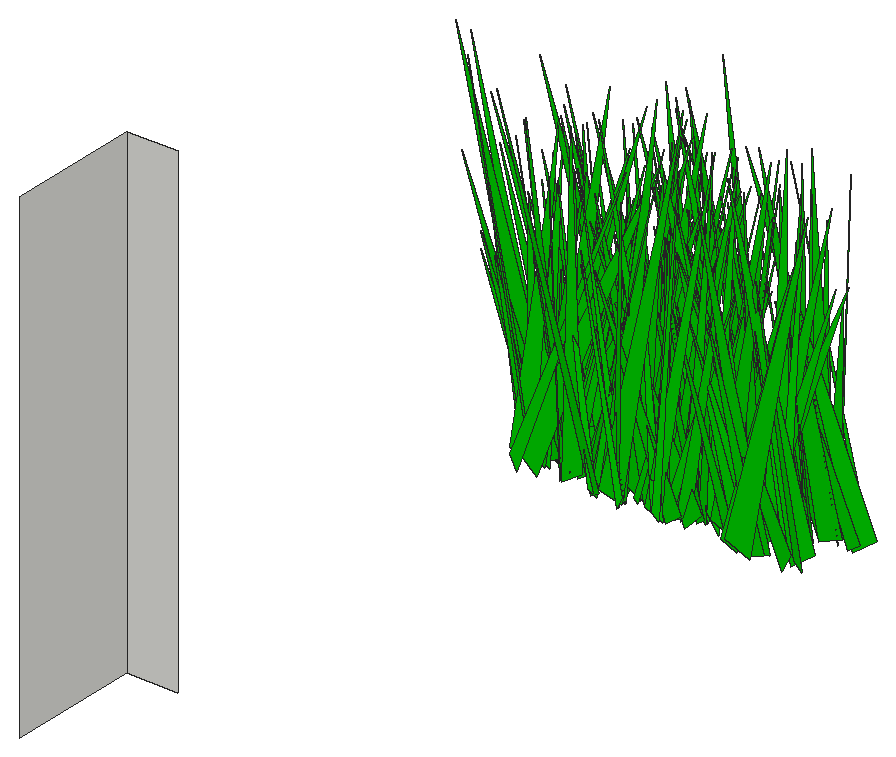
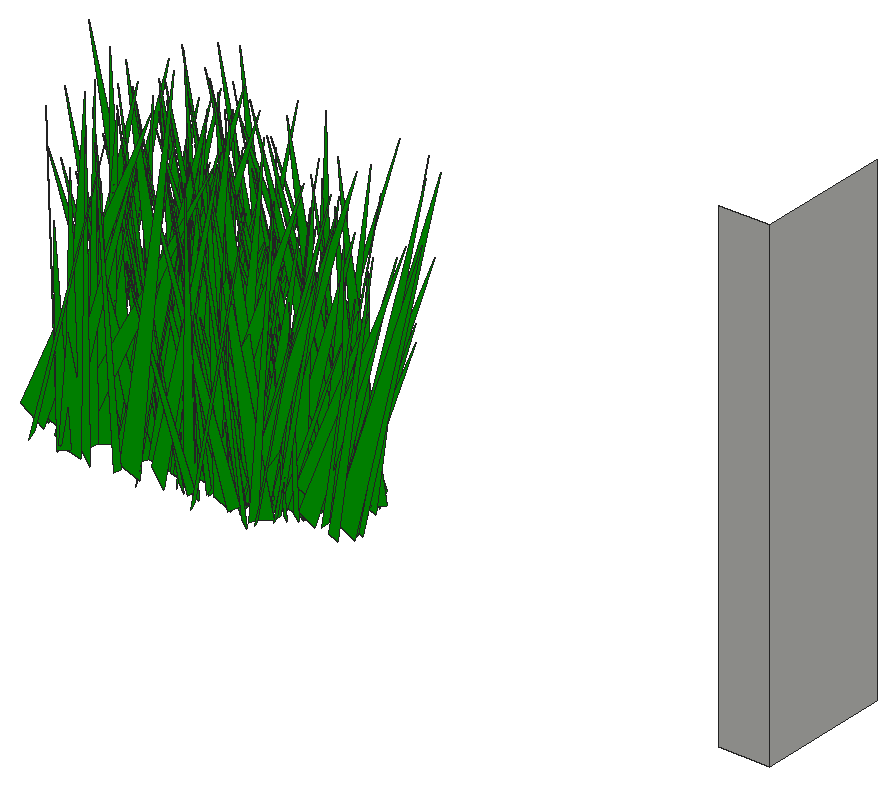
# SketchUp Ruby script. Lengths in inches.
U = 1.inch
M = Sketchup.active_model
def pt(a) = Geom::Point3d.new(a.map { |v| v * U })
def face(e, loops, mat)
  f = e.add_face(loops[0].map { |a| pt(a) })
  loops[1..].each { |l| e.add_face(l.map { |a| pt(a) }).erase! }
  f.material = f.back_material = mat if mat
  f
end
# faces: each face lists its corners as indices into pts; further lists are holes
def faces(e, pts, list, mat = nil) = list.each { |f| face(e, (f[0].is_a?(Array) ? f : [f]).map { |l| l.map { |i| pts[i] } }, mat) }
# xy, xz, yz: faces in a plane at the given z, y or x. An outline is a flat list of corners, or four numbers for a rectangle; further outlines are holes
def ring(l) = l.size == 4 ? [[l[0], l[1]], [l[2], l[1]], [l[2], l[3]], [l[0], l[3]]] : l.each_slice(2).to_a
def flat(e, list, mat, &to3) = list.each { |f| face(e, (f[0].is_a?(Array) ? f : [f]).map { |l| ring(l).map { |u, v| to3.(u, v) } }, mat) }
def xy(e, z, list, mat = nil) = flat(e, list, mat) { |x, y| [x, y, z] }
def xz(e, y, list, mat = nil) = flat(e, list, mat) { |x, z| [x, y, z] }
def yz(e, x, list, mat = nil) = flat(e, list, mat) { |y, z| [x, y, z] }
def lines(e, pts, list) = list.each { |a, b| e.add_line(pt(pts[a]), pt(pts[b])) }
# prism: a flat outline (further loops are holes) pulled along v
def prism(e, loops, v, mat = nil)
  f = face(e, loops, mat); d = Geom::Vector3d.new(v.map { |x| x * U })
  f.pushpull(f.normal.samedirection?(d) ? d.length : -d.length)
end
def box(e, o, s, mat = nil) = prism(e, [[o, [o[0] + s[0], o[1], o[2]], [o[0] + s[0], o[1] + s[1], o[2]], [o[0], o[1] + s[1], o[2]]]], [0, 0, s[2]], mat)
def at(x, y, z, deg = 0) = Geom::Transformation.translation(pt([x, y, z])) * Geom::Transformation.rotation(ORIGIN, Z_AXIS, deg.degrees)
def axes(o, x, y, z) = Geom::Transformation.new([*x, 0, *y, 0, *z, 0, *pt(o).to_a, 1])
def part(name) = M.definitions.add(name)
# library, detail: a bought-in or finely detailed component or shape, given as its bounding box
def library(name, o, s) = part(name).tap { |d| box(d.entities, o, s) }
def detail(e, o, s) = box(e.add_group.entities, o, s)
def put(e, d, t, mat = nil) = e.add_instance(d, t).tap { |i| i.material = mat if mat }
def group(e, t, mat = nil) = e.add_group.tap { |g| g.transformation = t; g.material = mat if mat }.entities
root = M.entities
M.materials.add("[Color G06]").color = [0, 204, 0]
c1 = part("fur_instance\#9")
p = [[0.8125,0,1.79],[0.67,-0.02,1.48],[0,-0.11,0],[0,0.11,0]]
faces(c1.entities,p,[[0,1,2,3]])
xz(root,8.54,[[0,-6,2.44,17.375]])
yz(root,0,[[2.125,-6,8.54,17.375]])
put(root,c1,axes([12.6,18.12,4.28],[-0.64533,0.75515,4.02371],[5.66112,-0.05738,3.26521],[-2.1274,-0.38176,7.46832]),"[Color G06]")
put(root,c1,axes([12.39,18.42,4.28],[-4.86092,0.42371,1.79988],[3.26268,0.64695,2.18743],[0.19462,-0.2629,8.28365]),"[Color G06]")
put(root,c1,axes([12.42,18.66,4.28],[-0.6628,-0.69624,0.76059],[-4.75092,0.06397,-2.52117],[-1.61763,0.0974,7.09297]),"[Color G06]")
put(root,c1,axes([13.09,16.5625,4.28],[-5.7551,0.03529,1.17459],[0.152,0.80381,-1.11066],[0.81153,0.09971,8.5378]),"[Color G06]")
put(root,c1,axes([12.39,19.37,4.28],[-4.0883,0.17136,1.83586],[1.50474,0.56814,1.39317],[0.86875,-0.17765,6.22637]),"[Color G06]")
put(root,c1,axes([13.73,17.02,4.28],[-2.9534,-0.5037,0.06023],[-3.46458,0.39291,-2.02157],[-1.02277,0.12356,6.67404]),"[Color G06]")
put(root,c1,axes([14.02,18.9,4.28],[-4.16734,0.4342,0.199],[3.0146,0.55371,2.22919],[-0.79087,-0.17731,7.44856]),"[Color G06]")
put(root,c1,axes([12.81,16.77,4.28],[-1.2675,-0.49753,1.55565],[-3.68712,0.14902,-1.23544],[-0.4678,0.17349,5.52256]),"[Color G06]")
put(root,c1,axes([13.4,16.95,4.28],[-2.71784,0.21877,0.15005],[1.50573,0.35423,1.59415],[-0.45173,-0.13546,4.41093]),"[Color G06]")
put(root,c1,axes([13.44,16.91,4.28],[-1.2543,-0.42644,1.06437],[-2.9311,0.12067,-2.16202],[-1.1261,0.16092,4.44191]),"[Color G06]")
put(root,c1,axes([13.64,18.1875,4.28],[-3.21131,0.39923,2.12033],[3.17906,0.37105,2.72946],[-0.32087,-0.31935,5.82193]),"[Color G06]")
put(root,c1,axes([12.95,16.74,4.28],[-0.19213,-0.40089,0.98908],[-2.83185,-0.00086,-1.26868],[-0.82685,0.09609,4.11523]),"[Color G06]")
put(root,c1,axes([13.23,18.79,4.28],[-3.53322,0.19435,0.6193],[1.29033,0.48908,-1.18747],[0.67021,0.08294,5.55105]),"[Color G06]")
put(root,c1,axes([13,17.03,4.28],[0.75321,0.54857,0.23993],[3.8591,-0.10738,1.1414],[-0.78031,-0.00154,5.87652]),"[Color G06]")
put(root,c1,axes([14.71,18.7,4.28],[-1.48296,0.4877,0.94635],[3.29219,0.15242,2.50041],[-1.33958,-0.16531,5.09742]),"[Color G06]")
put(root,c1,axes([13.66,18,4.28],[0.98697,0.61489,0.51583],[4.30032,-0.14494,1.46764],[-1.03464,-0.01585,6.59207]),"[Color G06]")
put(root,c1,axes([14.26,18.3,4.28],[-3.07882,-0.12929,0.02031],[-0.89322,0.4153,1.22464],[0.24885,-0.10888,4.64698]),"[Color G06]")
put(root,c1,axes([12.62,16.55,4.28],[-1.65023,0.71334,1.14507],[4.93889,0.25062,-2.03636],[1.53734,-0.03944,7.77119]),"[Color G06]")
put(root,c1,axes([14.11,17.19,4.28],[-3.77242,-0.57848,0.1182],[-4.02517,0.51385,1.92928],[1.0069,-0.11318,8.15528]),"[Color G06]")
put(root,c1,axes([13.32,16.78,4.28],[-2.61638,0.61188,0.04562],[4.14037,0.34588,-2.5034],[1.45345,0.11617,7.2134]),"[Color G06]")
put(root,c1,axes([15.03,16.41,4.28],[-4.78843,-0.09904,1.21671],[-0.86889,0.65957,-1.47084],[0.64204,0.15396,7.08387]),"[Color G06]")
put(root,c1,axes([15.09,19.31,4.28],[-4.8591,0.23305,0.0599],[1.50578,0.61759,-3.1786],[0.72625,0.2788,6.99117]),"[Color G06]")
put(root,c1,axes([15.18,18.91,4.28],[-3.17197,0.06794,0.34961],[0.54034,0.39502,2.13296],[-0.01014,-0.20166,4.29596]),"[Color G06]")
put(root,c1,axes([16.26,19.27,4.28],[-2.38032,-0.76955,0.75921],[-5.32677,0.29642,-2.79054],[-1.52931,0.16531,8.53807]),"[Color G06]")
put(root,c1,axes([15.75,18.04,4.28],[-2.96821,0.46373,1.60397],[3.45994,0.36251,2.26264],[-0.48957,-0.2496,6.26607]),"[Color G06]")
put(root,c1,axes([16.16,19.53,4.28],[-2.54932,0.61739,0.59802],[4.30336,0.3266,2.24535],[-1.11509,-0.15107,7.29809]),"[Color G06]")
put(root,c1,axes([14.08,17.01,4.28],[-1.56696,-0.3925,0.40315],[-2.67918,0.21984,1.32635],[0.90423,-0.02881,4.62852]),"[Color G06]")
put(root,c1,axes([16.65,15.95,4.28],[-5.39603,-0.33798,0.35312],[-2.42697,0.73976,-1.50508],[-0.20057,0.1415,8.71192]),"[Color G06]")
put(root,c1,axes([14.96,19.42,4.28],[-4.43034,-0.211,1.62602],[-1.33315,0.63221,1.31039],[1.30227,-0.07062,6.87321]),"[Color G06]")
put(root,c1,axes([12.61,17.81,4.28],[3.89225,0.27465,0.68493],[2.01617,-0.51637,-1.80693],[0.15599,-0.17898,6.26425]),"[Color G06]")
put(root,c1,axes([16.0625,18.89,4.28],[-2.86827,-0.54522,1.56949],[-4.0037,0.3554,-2.16157],[-0.60029,0.23476,6.91754]),"[Color G06]")
put(root,c1,axes([16.22,19.51,4.28],[-4.872,0.30301,1.23864],[2.32125,0.65009,2.12558],[0.14323,-0.22866,7.68443]),"[Color G06]")
put(root,c1,axes([15.85,19.6,4.28],[-1.81565,-0.59536,0.8356],[-4.23613,0.2318,-1.58835],[-0.77208,0.12825,6.74969]),"[Color G06]")
put(root,c1,axes([14.73,18.76,4.28],[1.42496,-0.67391,0.91843],[-4.77584,-0.21086,-1.22244],[-0.96183,0.04861,7.43055]),"[Color G06]")
put(root,c1,axes([14.85,16.08,4.28],[-4.09742,-0.045,2.33983],[-0.63064,0.59746,-1.14674],[1.46881,0.13098,6.03488]),"[Color G06]")
put(root,c1,axes([15.32,20.39,4.28],[-3.07333,-0.12945,0.46687],[-0.83142,0.42063,1.17171],[0.51773,-0.09293,4.65302]),"[Color G06]")
put(root,c1,axes([13.43,16.62,4.28],[3.7685,0.34962,1.73775],[2.72815,-0.51443,-1.32619],[-0.44179,-0.19443,6.63366]),"[Color G06]")
put(root,c1,axes([13.4375,17.25,4.28],[1.62705,-0.41864,2.04455],[-3.24418,-0.16434,1.90124],[0.59992,0.24669,4.73624]),"[Color G06]")
put(root,c1,axes([13.625,17.37,4.28],[-1.83862,0.79986,1.31914],[5.43881,0.28253,-2.74599],[2.02488,-0.03258,8.57351]),"[Color G06]")
put(root,c1,axes([14.43,19.05,4.28],[3.13799,-0.14184,1.23323],[-0.72732,-0.43713,-1.64163],[-1.08927,-0.11674,4.64886]),"[Color G06]")
put(root,c1,axes([15.46,16.75,4.28],[1.77986,0.44421,0.90069],[2.95757,-0.26174,1.77383],[-1.32809,0.01244,5.15729]),"[Color G06]")
put(root,c1,axes([14.97,16.74,4.28],[3.72768,-0.33079,1.95353],[-2.23798,-0.55084,-1.17566],[-1.52552,-0.00021,6.49824]),"[Color G06]")
put(root,c1,axes([14.7,19.38,4.28],[2.70692,-0.06976,0.94677],[-0.30426,-0.37451,-1.22653],[-0.74763,-0.10015,3.9271]),"[Color G06]")
put(root,c1,axes([14.01,17.6875,4.28],[3.27522,-0.04761,0.47283],[-0.40922,-0.44394,1.19629],[-0.22184,0.11596,4.77398]),"[Color G06]")
put(root,c1,axes([12.93,17.09,4.28],[1.91813,0.69062,2.01417],[4.87371,-0.18215,-3.19302],[1.60975,-0.27144,7.26725]),"[Color G06]")
put(root,c1,axes([15.51,20.28,4.28],[-4.11225,-0.35239,1.60412],[-2.29893,0.5893,1.70698],[1.50104,-0.06287,7.00896]),"[Color G06]")
put(root,c1,axes([12.75,17.93,4.28],[4.19638,-0.62533,0.46819],[-4.41144,-0.56136,2.19177],[0.86432,0.17088,8.91357]),"[Color G06]")
put(root,c1,axes([12.74,15.92,4.28],[5.5787,-0.15719,0.28304],[-1.1038,-0.70664,3.51468],[0.29698,0.32637,7.74621]),"[Color G06]")
put(root,c1,axes([15.19,16.39,4.28],[4.11185,-0.5843,0.79358],[-3.91118,-0.56575,-2.58402],[-1.59446,-0.11905,8.38505]),"[Color G06]")
put(root,c1,axes([16.32,18.85,4.28],[0.9565,-0.52741,2.39794],[-3.85514,-0.19463,-1.48238],[-1.42016,0.17311,5.63911]),"[Color G06]")
put(root,c1,axes([14.11,17.9,4.28],[3.17358,-0.39234,1.286],[-2.93957,-0.41531,1.64866],[0.12501,0.1943,6.12066]),"[Color G06]")
put(root,c1,axes([16.49,15.97,4.28],[-4.24399,0.24039,0.79583],[1.59749,0.58886,-1.40351],[0.83864,0.09479,6.70085]),"[Color G06]")
put(root,c1,axes([13.86,18.06,4.28],[3.76419,-0.44504,0.8697],[-3.23233,-0.50393,1.62728],[0.27609,0.16779,7.19404]),"[Color G06]")
put(root,c1,axes([13.35,18.18,4.28],[3.60775,0.39463,0.19663],[2.50258,-0.43,-3.43109],[1.32786,-0.26178,5.93223]),"[Color G06]")
put(root,c1,axes([13.1,16.26,4.28],[2.78587,0.74928,0.24398],[4.9022,-0.34357,-3.8275],[2.20627,-0.18274,8.19638]),"[Color G06]")
put(root,c1,axes([15.64,20.66,4.28],[2.77205,-0.13604,0.2967],[-0.84998,-0.36604,-1.54058],[-0.51833,-0.12729,4.11306]),"[Color G06]")
put(root,c1,axes([17.41,16.62,4.28],[-4.96591,0.02105,2.38419],[0.87829,0.64164,3.43557],[1.3402,-0.3425,6.58274]),"[Color G06]")
put(root,c1,axes([15.28,19.92,4.28],[2.28876,-0.5763,1.14703],[-4.17279,-0.29681,1.46812],[0.5069,0.15881,6.90643]),"[Color G06]")
put(root,c1,axes([19.11,18.54,4.28],[-3.26037,0.62882,0.15228],[4.33887,0.43243,2.37865],[-1.23275,-0.14109,7.96933]),"[Color G06]")
put(root,c1,axes([17.69,17.83,4.28],[-3.57023,0.21524,0.11924],[1.45627,0.47783,-1.68617],[0.51789,0.14021,5.56341]),"[Color G06]")
put(root,c1,axes([16.46,19.25,4.28],[-3.02344,0.38324,0.71382],[2.23871,0.39196,-2.9928],[1.66415,0.16898,5.32296]),"[Color G06]")
put(root,c1,axes([17.66,16.39,4.28],[-3.50206,-0.14153,0.48361],[-0.86546,0.46841,1.74738],[0.62109,-0.14531,5.16171]),"[Color G06]")
put(root,c1,axes([18.01,20.8,4.28],[-4.67944,-0.20343,0.79254],[-1.26022,0.63501,2.10365],[0.9063,-0.16739,7.01724]),"[Color G06]")
put(root,c1,axes([17.82,15.96,4.28],[-3.69863,0.04728,1.40876],[0.65085,0.49563,1.90616],[0.76146,-0.19399,5.21351]),"[Color G06]")
put(root,c1,axes([16.61,16.66,4.28],[4.18489,0.02655,2.10438],[-0.08895,-0.60463,1.27157],[-1.41805,0.11629,6.13062]),"[Color G06]")
put(root,c1,axes([16.14,16.7,4.28],[4.44378,-0.07949,1.7674],[-0.89846,-0.60852,1.90223],[-0.95713,0.20218,6.42009]),"[Color G06]")
put(root,c1,axes([17.51,18.98,4.28],[4.52933,-0.58651,0.90492],[-3.46216,-0.58088,-4.54135],[-2.46391,-0.26194,8.04475]),"[Color G06]")
put(root,c1,axes([17.34,19.83,4.28],[-2.79905,0.02637,2.21928],[0.8092,0.39605,1.73908],[1.25931,-0.19587,3.81526]),"[Color G06]")
put(root,c1,axes([18.38,17.66,4.28],[0.19152,-0.5431,1.40616],[-3.82701,-0.06369,-1.66157],[-1.18655,0.11777,5.58607]),"[Color G06]")
put(root,c1,axes([15.85,19.15,4.28],[1.58108,0.49581,0.41329],[3.42313,-0.19916,-1.80632],[1.00031,-0.10214,5.52812]),"[Color G06]")
put(root,c1,axes([18.76,16.87,4.28],[-0.23775,-0.64823,0.80236],[-4.48704,0.0103,-2.01398],[-1.32844,0.08122,6.65895]),"[Color G06]")
put(root,c1,axes([17.97,19.17,4.28],[-4.0406,0.42406,0.02882],[2.71146,0.50439,-3.38817],[1.377,0.25114,6.75624]),"[Color G06]")
put(root,c1,axes([16.45,19.46,4.28],[1.36358,-0.31561,1.13591],[-2.29855,-0.14053,1.67817],[0.64574,0.16625,3.57489]),"[Color G06]")
put(root,c1,axes([16.65,19.22,4.28],[-1.14858,-0.51583,1.97946],[-3.59211,0.21582,1.80491],[1.59205,0.11481,5.50047]),"[Color G06]")
put(root,c1,axes([16.23,18.91,4.28],[-1.40892,-0.82224,1.31858],[-5.54784,0.2271,3.02667],[2.18366,0.04646,8.54035]),"[Color G06]")
put(root,c1,axes([16.33,19.89,4.28],[4.60776,0.23037,1.65594],[1.90798,-0.62209,-1.91749],[-0.56254,-0.22299,7.06013]),"[Color G06]")
put(root,c1,axes([15.77,17.31,4.28],[6.06197,0.03651,0.75718],[0.15253,-0.8306,1.87272],[-0.54949,0.17219,8.87303]),"[Color G06]")
put(root,c1,axes([15.8125,16.52,4.28],[5.7048,0.10241,0.87075],[0.83648,-0.78227,-1.67315],[-0.42312,-0.1658,8.43221]),"[Color G06]")
put(root,c1,axes([19.18,18.16,4.28],[-2.03536,0.46425,0.74775],[3.30557,0.26013,1.54613],[-0.63822,-0.13325,5.62331]),"[Color G06]")
put(root,c1,axes([17.47,16.18,4.28],[-3.91247,-0.34174,2.19717],[-1.91339,0.57139,2.59865],[2.12279,-0.11483,6.39188]),"[Color G06]")
put(root,c1,axes([17.29,19.93,4.28],[4.10563,-0.474,0.3554],[-3.20249,-0.55449,-2.31498],[-1.16403,-0.1463,7.62253]),"[Color G06]")
put(root,c1,axes([16.5,18.76,4.28],[0.94972,0.78231,1.6787],[5.57701,-0.09112,-2.16961],[1.27765,-0.18376,8.22267]),"[Color G06]")
put(root,c1,axes([19.55,16.65,4.28],[-5.18526,0.28858,2.44451],[2.54447,0.67984,2.83657],[0.69551,-0.33564,7.84726]),"[Color G06]")
put(root,c1,axes([17.22,16.31,4.28],[1.77138,0.79213,2.26926],[5.87396,-0.22837,-1.0845],[0.2663,-0.2317,8.82688]),"[Color G06]")
put(root,c1,axes([17.43,18.36,4.28],[5.04773,0.11169,2.81533],[1.45584,-0.68725,-2.69868],[-1.43888,-0.30354,7.14598]),"[Color G06]")
put(root,c1,axes([15.83,16.86,4.28],[4.16113,0.60438,1.18707],[4.3419,-0.53643,-2.62314],[0.75101,-0.24738,8.58826]),"[Color G06]")
put(root,c1,axes([18.56,18,4.28],[-3.82504,0.26552,1.60154],[1.6768,0.54988,-1.52667],[1.40077,0.0668,6.20078]),"[Color G06]")
put(root,c1,axes([20.1875,16.25,4.28],[-1.18163,-0.49068,1.02179],[-3.2458,0.10386,-2.65503],[-1.52126,0.15954,4.87116]),"[Color G06]")
put(root,c1,axes([20.87,16.58,4.28],[-1.5268,-0.56849,2.21715],[-3.78556,0.06746,-3.83606],[-2.11912,0.28908,5.25525]),"[Color G06]")
put(root,c1,axes([19.57,18.86,4.28],[-0.18153,0.84696,0.75523],[5.97547,0.01085,1.81002],[-1.1999,-0.07408,8.89955]),"[Color G06]")
put(root,c1,axes([16.8,18.07,4.28],[3.47396,-0.24434,0.15266],[-1.68974,-0.45703,1.86186],[0.47481,0.16123,5.50903]),"[Color G06]")
put(root,c1,axes([17.02,19.81,4.28],[4.74234,0.18608,0.87204],[1.41708,-0.65353,-1.19397],[-0.33632,-0.12973,7.26559]),"[Color G06]")
put(root,c1,axes([17.96,17.95,4.28],[3.79081,-0.18355,0.87348],[-1.11047,-0.51863,-1.75471],[-0.91712,-0.13073,5.73506]),"[Color G06]")
put(root,c1,axes([16.71,17.24,4.28],[0.34699,0.64805,2.40974],[4.47524,0.05197,-3.04507],[2.04196,-0.22403,6.26423]),"[Color G06]")
put(root,c1,axes([18.69,20.05,4.28],[2.86106,0.52154,1.41685],[3.63867,-0.41945,1.32394],[-1.28339,-0.02656,6.91219]),"[Color G06]")
put(root,c1,axes([18.34,17.21,4.28],[4.70981,0.30875,2.1134],[1.97475,-0.68302,1.63232],[-1.73269,0.0608,7.60499]),"[Color G06]")
put(root,c1,axes([17.87,16.92,4.28],[-1.68137,-0.69161,1.49515],[-4.76217,0.26598,2.17118],[1.70926,0.06072,7.5199]),"[Color G06]")
put(root,c1,axes([20.41,19.92,4.28],[-4.80742,-0.35088,2.47146],[-2.99409,0.60307,-3.17376],[0.31875,0.37267,7.46295]),"[Color G06]")
put(root,c1,axes([16.67,20.02,4.28],[4.43511,-0.29988,0.12527],[-2.12147,-0.60467,1.49321],[0.36211,0.13037,7.21382]),"[Color G06]")
put(root,c1,axes([17.5,17.85,4.28],[1.01531,0.54547,0.1083],[3.77974,-0.13406,-1.58638],[1.00999,-0.04663,5.82797]),"[Color G06]")
put(root,c1,axes([19.52,16.07,4.28],[-3.33423,0.34048,0.16892],[2.29563,0.44535,-1.90323],[0.8394,0.13446,5.87602]),"[Color G06]")
put(root,c1,axes([17.2,16.16,4.28],[3.87574,-0.63727,1.4449],[-4.66767,-0.52155,1.54267],[0.18143,0.19558,8.82196]),"[Color G06]")
put(root,c1,axes([18.23,19.5625,4.28],[3.71057,-0.02031,1.38985],[-0.325,-0.52259,1.06092],[-0.88338,0.10695,5.44764]),"[Color G06]")
put(root,c1,axes([18.17,17.39,4.28],[-0.1145,-0.67095,2.26635],[-4.95834,0.05397,1.27587],[0.93029,0.20507,7.07921]),"[Color G06]")
put(root,c1,axes([19.56,19.47,4.28],[1.08603,-0.52078,1.35757],[-3.67637,-0.17915,-1.32504],[-1.12117,0.08297,5.6599]),"[Color G06]")
put(root,c1,axes([16.23,18.51,4.28],[4.51889,0.44702,0.83562],[3.07672,-0.54349,-3.76695],[1.05961,-0.32828,7.37421]),"[Color G06]")
put(root,c1,axes([18.59,18.24,4.28],[3.22046,-0.10344,1.10682],[-0.51888,-0.44724,-1.42898],[-0.91073,-0.11096,4.72801]),"[Color G06]")
put(root,c1,axes([21.04,17.62,4.28],[-1.43706,-0.5105,1.53429],[-3.47752,0.1146,-2.89539],[-1.53729,0.21798,5.11544]),"[Color G06]")
put(root,c1,axes([17.89,17.02,4.28],[4.11444,0.15682,1.49032],[1.4135,-0.54149,-2.17125],[-0.51099,-0.23515,5.99376]),"[Color G06]")
put(root,c1,axes([19.49,17.17,4.28],[0.92521,0.64676,0.28265],[4.56531,-0.13165,1.22345],[-0.83986,-0.00312,6.96182]),"[Color G06]")
put(root,c1,axes([20.16,18.32,4.28],[-4.51396,-0.21759,0.28068],[-1.27298,0.55289,3.50661],[0.92173,-0.302,6.21746]),"[Color G06]")
put(root,c1,axes([19.9,19.42,4.28],[-5.09034,0.19602,2.83713],[1.76823,0.73319,1.26742],[1.56618,-0.19067,7.79023]),"[Color G06]")
put(root,c1,axes([21.0625,16.78,4.28],[-3.85699,-0.28543,0.79142],[-2.11422,0.51974,-1.48315],[-0.01309,0.15684,6.35524]),"[Color G06]")
put(root,c1,axes([21.08,18.9,4.28],[-4.10035,-0.03906,0.28357],[-0.32535,0.54354,-1.90699],[0.09288,0.17941,5.83904]),"[Color G06]")
put(root,c1,axes([19.74,16.62,4.28],[-3.7907,0.04679,2.1092],[0.01711,0.55203,-1.33797],[1.45048,0.11576,5.52802]),"[Color G06]")
put(root,c1,axes([18.05,19.45,4.28],[2.2937,0.36132,1.42844],[2.68612,-0.25159,-2.32412],[0.64204,-0.23826,4.62035]),"[Color G06]")
put(root,c1,axes([18.15,16.53,4.28],[3.70183,-0.05844,0.30451],[-0.45399,-0.5036,1.22518],[-0.10513,0.11687,5.43153]),"[Color G06]")
put(root,c1,axes([19.55,16.29,4.28],[-2.4615,0.46949,0.98331],[3.22619,0.3552,-1.44205],[1.16629,0.00834,6.06431]),"[Color G06]")
put(root,c1,axes([20.41,17.42,4.28],[1.30204,0.68496,0.06509],[4.68824,-0.17515,2.25072],[-1.46637,0.0482,7.25374]),"[Color G06]")
put(root,c1,axes([19.73,19.56,4.28],[-4.50566,-0.23023,1.96719],[-0.71041,0.5726,4.0638],[1.9884,-0.31712,5.90949]),"[Color G06]")
put(root,c1,axes([20.89,17.3125,4.28],[-1.77429,-0.52717,0.95638],[-3.8118,0.23191,-1.11216],[-0.41397,0.12409,6.14161]),"[Color G06]")
put(root,c1,axes([22.42,17.375,4.28],[0.13061,0.77434,3.36502],[5.26746,-0.16454,3.89277],[-2.85642,-0.26801,7.33243]),"[Color G06]")
put(root,c1,axes([21.15,17.23,4.28],[-4.84362,0.0031,1.29725],[0.24966,0.66197,1.90028],[0.83159,-0.18066,6.98537]),"[Color G06]")
put(root,c1,axes([18.21,17.73,4.28],[4.05647,0.55084,1.08162],[4.01481,-0.55278,-1.29418],[0.09665,-0.15679,8.36286]),"[Color G06]")
put(root,c1,axes([19.52,16,4.28],[4.92094,-0.04428,2.84782],[-0.80804,-0.70766,1.85488],[-1.7546,0.20171,7.13276]),"[Color G06]")
put(root,c1,axes([20.3125,17.14,4.28],[-3.08825,0.46477,0.98212],[3.19047,0.43934,-1.47382],[1.16684,0.02882,6.62918]),"[Color G06]")
put(root,c1,axes([20.94,18.26,4.28],[-5.26309,0.04428,2.26148],[-0.3613,0.69267,-3.43617],[1.50328,0.3215,7.09176]),"[Color G06]")
put(root,c1,axes([19.98,18.1875,4.28],[4.2731,0.02003,2.50784],[0.44456,-0.62892,-1.1151],[-1.62436,-0.11944,6.29202]),"[Color G06]")
put(root,c1,axes([21,20.37,4.28],[-4.45461,-0.22791,0.52269],[-1.16734,0.52359,4.00366],[1.19621,-0.33777,5.85347]),"[Color G06]")
put(root,c1,axes([22.15,19.65,4.28],[-2.88772,-0.76387,0.5406],[-5.43225,0.38936,-1.61772],[-0.79305,0.11444,9.11259]),"[Color G06]")
put(root,c1,axes([18.65,20.08,4.28],[2.81383,0.27003,0.17259],[1.86724,-0.36932,-1.62328],[0.52589,-0.13349,4.84016]),"[Color G06]")
put(root,c1,axes([19.4,17,4.28],[2.60692,0.37314,1.61725],[2.88199,-0.34771,-1.16114],[-0.15924,-0.18442,5.46138]),"[Color G06]")
put(root,c1,axes([20.34,18.08,4.28],[3.298,-0.4156,1.01243],[-2.66096,-0.4588,-2.27276],[-1.50361,-0.09963,6.24278]),"[Color G06]")
put(root,c1,axes([21,19.17,4.28],[0.69321,-0.55048,1.062],[-3.87046,-0.11819,-1.39429],[-1.05269,0.07206,5.82575]),"[Color G06]")
put(root,c1,axes([19.95,18.46,4.28],[4.22287,-0.49658,0.47269],[-3.25687,-0.56249,-2.88866],[-1.47452,-0.17974,7.7341]),"[Color G06]")
put(root,c1,axes([19.25,19.95,4.28],[3.53319,-0.09592,0.0898],[-0.58145,-0.43688,-2.50377],[-0.37237,-0.22791,4.76161]),"[Color G06]")
put(root,c1,axes([19.53,18.26,4.28],[5.12713,0.21612,1.47221],[1.25939,-0.71028,2.18084],[-1.33654,0.15979,7.70254]),"[Color G06]")
put(root,c1,axes([21.5,20.25,4.28],[2.9979,0.62169,4.75975],[4.8523,-0.53635,1.22082],[-2.5444,-0.29035,7.93627]),"[Color G06]")
put(root,c1,axes([19.78,17,4.28],[0.87839,0.40549,1.55174],[3.02537,-0.08294,-1.33562],[0.61711,-0.17054,4.33908]),"[Color G06]")
put(root,c1,axes([19.24,16.16,4.28],[5.03333,-0.36131,2.1263],[-2.87983,-0.68772,1.80327],[-0.66645,0.24296,8.26651]),"[Color G06]")
put(root,c1,axes([22.83,17.85,4.28],[-3.19365,0.69826,1.34868],[5.03106,0.41119,2.15625],[-0.75964,-0.21234,8.61065]),"[Color G06]")
put(root,c1,axes([19.61,17.14,4.28],[-0.26367,0.70518,2.97373],[5.14988,0.12113,-2.27961],[1.73534,-0.25231,7.21694]),"[Color G06]")
put(root,c1,axes([23.48,16.62,4.28],[-2.92372,0.72717,1.39569],[5.12762,0.35104,2.9832],[-1.33168,-0.24484,8.42253]),"[Color G06]")
put(root,c1,axes([20.04,17.71,4.28],[1.40393,0.398,0.73048],[2.83494,-0.17348,-1.31266],[0.59001,-0.11347,4.56903]),"[Color G06]")
put(root,c1,axes([21.12,17.88,4.28],[-2.79158,-0.36912,1.28455],[-2.41607,0.40567,1.66272],[1.38138,-0.0364,5.50404]),"[Color G06]")
put(root,c1,axes([20.45,16.82,4.28],[5.23621,-0.39126,1.17382],[-2.52997,-0.72227,-2.44608],[-1.4452,-0.15319,8.53503]),"[Color G06]")
put(root,c1,axes([19.72,16.47,4.28],[3.68943,-0.18773,0.50128],[-1.38551,-0.49162,1.62889],[0.07225,0.15869,5.6392]),"[Color G06]")
put(root,c1,axes([19.5,18.14,4.28],[5.24545,-0.11191,0.41175],[-0.76001,-0.72664,-1.06055],[-0.37735,-0.09219,7.85971]),"[Color G06]")
put(root,c1,axes([24.87,19.38,4.28],[-5.4232,-0.42469,0.43155],[-2.68201,0.62062,-5.12725],[-1.47159,0.434,7.75418]),"[Color G06]")
put(root,c1,axes([21.02,16.95,4.28],[3.17576,0.22848,2.38841],[2.04393,-0.45462,-1.07482],[-1.02992,-0.19771,5.23163]),"[Color G06]")
put(root,c1,axes([20.26,19.08,4.28],[2.58834,0.40224,1.0046],[2.95279,-0.3407,-1.32326],[0.23178,-0.1516,5.63921]),"[Color G06]")
put(root,c1,axes([22.91,16.34,4.28],[-2.45312,-0.30756,0.47434],[-2.1878,0.31995,-1.44301],[-0.42283,0.12887,4.71446]),"[Color G06]")
put(root,c1,axes([23.09,17.11,4.28],[1.67774,-0.63615,1.71612],[-4.0092,-0.28229,-3.26529],[-2.46097,0.02619,6.48948]),"[Color G06]")
put(root,c1,axes([23.44,17.63,4.28],[-3.18056,0.46292,1.65856],[3.45421,0.38128,2.57157],[-0.56618,-0.27437,6.37188]),"[Color G06]")
put(root,c1,axes([22.33,17.93,4.28],[1.05222,0.34059,1.64417],[2.39628,-0.19334,1.17518],[-1.19728,-0.08764,3.79702]),"[Color G06]")
put(root,c1,axes([20.39,16.6,4.28],[4.39465,-0.38576,0.03238],[-2.71934,-0.60339,-1.37616],[-0.50858,-0.10708,7.63815]),"[Color G06]")
put(root,c1,axes([21.48,16.97,4.28],[-4.91331,0.45996,1.7323],[2.44299,0.65109,-4.38172],[2.50109,0.26762,7.683]),"[Color G06]")
put(root,c1,axes([23.67,17.66,4.28],[-2.23855,0.45299,0.31346],[3.14205,0.29139,1.74868],[-0.85113,-0.11571,5.63102]),"[Color G06]")
put(root,c1,axes([23.24,17.33,4.28],[-4.90645,0.11667,0.99137],[0.64861,0.67123,-1.90365],[0.8481,0.1616,7.19119]),"[Color G06]")
put(root,c1,axes([24.03,17.15,4.28],[-3.39674,0.38413,0.41005],[2.68905,0.44344,2.03707],[-0.65772,-0.17081,6.21075]),"[Color G06]")
put(root,c1,axes([22.91,18.73,4.28],[0.27553,-0.43497,0.03245],[-2.93318,-0.03716,-1.59008],[-1.0616,-0.01022,4.40179]),"[Color G06]")
put(root,c1,axes([22.91,18.52,4.28],[0.771,-0.6582,1.07174],[-4.60876,-0.12905,-1.69814],[-1.24617,0.07003,6.9434]),"[Color G06]")
put(root,c1,axes([21.18,18.41,4.28],[1.88844,0.27501,0.98893],[2.06748,-0.23435,-1.33243],[0.23001,-0.15146,3.85732]),"[Color G06]")
put(root,c1,axes([20.86,18.02,4.28],[1.30216,-0.74581,2.04371],[-5.43582,-0.13905,1.90728],[0.96294,0.2236,8.00298]),"[Color G06]")
put(root,c1,axes([21.46,18.27,4.28],[5.1219,0.08753,1.69682],[0.26143,-0.70121,2.39235],[-1.27067,0.20854,7.33189]),"[Color G06]")
put(root,c1,axes([21.62,18.05,4.28],[4.73568,0.49426,0.42115],[3.33606,-0.64028,2.52643],[-1.23025,0.16636,8.47209]),"[Color G06]")
put(root,c1,axes([24.16,16.42,4.28],[-2.37869,0.35154,0.58001],[2.42047,0.28776,2.13844],[-0.8046,-0.17363,4.71832]),"[Color G06]")
put(root,c1,axes([23.91,17.99,4.28],[-2.48221,-0.56559,1.43559],[-4.14861,0.32014,-1.53393],[-0.40352,0.18777,6.93959]),"[Color G06]")
put(root,c1,axes([21.9,20.47,4.28],[-3.61496,-0.32172,3.13396],[-2.0365,0.58267,1.62396],[2.3606,0.01,6.20026]),"[Color G06]")
put(root,c1,axes([25.58,16.32,4.28],[-4.15897,-0.36626,0.57843],[-2.36101,0.46437,-4.14226],[-1.21414,0.35159,6.07363]),"[Color G06]")
put(root,c1,axes([24.32,16.26,4.28],[-1.71597,-0.69308,0.31496],[-4.9295,0.23271,-1.16487],[-0.66931,0.06297,7.77187]),"[Color G06]")
put(root,c1,axes([23.15,17.4375,4.28],[2.66823,0.17988,0.97482],[0.80754,-0.34386,2.35178],[-1.19891,0.16873,3.75358]),"[Color G06]")
put(root,c1,axes([21.375,17.52,4.28],[3.74145,-0.3628,0.08104],[-2.57672,-0.51463,1.06845],[0.3642,0.08611,6.72667]),"[Color G06]")
put(root,c1,axes([24.33,16.1,4.28],[-1.41226,-0.44337,0.47842],[-3.13995,0.18346,-1.17297],[-0.59369,0.08435,5.06566]),"[Color G06]")
put(root,c1,axes([24.91,20.06,4.28],[-3.97659,0.33806,1.65507],[2.66521,0.5022,2.52034],[-0.02091,-0.28131,6.48842]),"[Color G06]")
put(root,c1,axes([22.05,16.875,4.28],[0.15866,-0.73927,0.16323],[-5.14224,-0.01773,1.93968],[1.29434,0.02018,7.68607]),"[Color G06]")
put(root,c1,axes([23.94,16.49,4.28],[3.93861,0.59399,1.07547],[3.5535,-0.52268,4.09263],[-2.45667,0.19627,7.64412]),"[Color G06]")
put(root,c1,axes([21.625,19.12,4.28],[2.59062,-0.45967,0.63287],[-3.23811,-0.33224,1.88732],[0.74841,0.15363,5.97509]),"[Color G06]")
put(root,c1,axes([23.58,16.82,4.28],[2.16933,0.32334,0.80134],[2.04945,-0.30523,1.75488],[-1.2099,0.06272,4.40936]),"[Color G06]")
put(root,c1,axes([23.67,19.15,4.28],[-2.15025,0.52715,0.2627],[3.69526,0.29855,-1.25633],[0.81653,0.0371,6.37742]),"[Color G06]")
put(root,c1,axes([23.43,20.46,4.28],[4.66681,-0.26103,1.93113],[-1.31989,-0.64571,-2.90149],[-1.85245,-0.19754,6.93238]),"[Color G06]")
put(root,c1,axes([24.99,18.27,4.28],[-4.38616,-0.10403,1.41655],[-1.0717,0.56483,-2.64742],[0.55345,0.2693,6.09984]),"[Color G06]")
put(root,c1,axes([24.37,18.28,4.28],[0.78816,0.71385,0.6802],[5.04911,-0.11953,1.34191],[-0.95902,-0.04265,7.62396]),"[Color G06]")
put(root,c1,axes([23.84,19.55,4.28],[-4.34691,-0.43453,2.28372],[-2.74198,0.63934,2.31614],[2.12762,-0.06384,7.65076]),"[Color G06]")
put(root,c1,axes([24.26,20.42,4.28],[2.6689,-0.6253,2.23591],[-4.48247,-0.41084,-1.24691],[-1.50109,0.11506,7.69883]),"[Color G06]")
put(root,c1,axes([24.02,17.6,4.28],[-2.85844,0.73097,1.07764],[5.11518,0.41097,-1.71585],[1.35401,-0.00943,8.75712]),"[Color G06]")
put(root,c1,axes([25.79,18.7,4.28],[-2.30304,-0.69255,2.15745],[-5.10292,0.26838,-2.27139],[-0.84245,0.26764,7.86038]),"[Color G06]")
put(root,c1,axes([23.03,16.04,4.28],[0.88935,0.4944,0.80835],[3.48626,-0.10093,-1.4766],[0.84203,-0.10431,5.25983]),"[Color G06]")
put(root,c1,axes([27.1,19.14,4.28],[-3.10084,0.71069,0.80643],[4.77088,0.36816,3.70627],[-1.87208,-0.23893,8.10944]),"[Color G06]")
put(root,c1,axes([24.3125,20.2,4.28],[2.34384,0.52696,0.9849],[3.64874,-0.3395,1.47047],[-1.18397,-0.00305,6.48143]),"[Color G06]")
put(root,c1,axes([26.17,20.32,4.28],[-5.3435,0.11099,0.15838],[0.75646,0.72918,-1.69177],[0.26929,0.15402,7.89515]),"[Color G06]")
put(root,c1,axes([25.96,16.82,4.28],[2.07059,-0.75561,1.9008],[-4.85955,-0.33768,-3.59561],[-2.71375,0.02815,7.889]),"[Color G06]")
put(root,c1,axes([25.3,18.22,4.28],[-4.04417,0.01266,1.30122],[-0.07842,0.56634,-1.17736],[0.87183,0.10966,5.93008]),"[Color G06]")
put(root,c1,axes([23.46,16.4375,4.28],[1.47536,-0.46368,1.40724],[-3.42935,-0.17877,1.26463],[0.42753,0.16615,5.28779]),"[Color G06]")
put(root,c1,axes([22.97,18.34,4.28],[2.46549,0.64192,0.80296],[4.60397,-0.32948,-1.31922],[0.53221,-0.12351,7.69244]),"[Color G06]")
put(root,c1,axes([25.27,16.69,4.28],[-3.26989,-0.00411,1.14573],[0.17552,0.45158,1.3051],[0.74681,-0.12413,4.70982]),"[Color G06]")
put(root,c1,axes([24.42,17.52,4.28],[-4.56776,0.39379,1.67397],[1.99655,0.60168,-4.09034],[2.28981,0.26093,6.90573]),"[Color G06]")
put(root,c1,axes([23.03,18.12,4.28],[1.21994,0.57224,0.33927],[3.91572,-0.1518,-2.03959],[1.24861,-0.08306,6.06478]),"[Color G06]")
put(root,c1,axes([22.63,18.48,4.28],[2.18635,0.52507,1.27753],[3.6131,-0.2299,-2.95779],[1.36179,-0.23303,5.79654]),"[Color G06]")
put(root,c1,axes([24.49,20.47,4.28],[-1.10541,-0.478,0.20962],[-3.29043,0.15353,1.459],[0.97122,-0.02389,5.18155]),"[Color G06]")
put(root,c1,axes([26.85,18.82,4.28],[-2.18564,-0.42301,0.1731],[-2.82884,0.27658,-2.14326],[-1.10152,0.12905,5.16068]),"[Color G06]")
put(root,c1,axes([26.0625,18.79,4.28],[-3.5824,0.00595,0.65792],[-0.09911,0.47745,-1.70155],[0.43102,0.15925,5.077]),"[Color G06]")
put(root,c1,axes([26.12,19.0625,4.28],[-0.58825,-0.40177,1.08141],[-2.85027,0.04735,-1.44258],[-0.83719,0.12111,4.15153]),"[Color G06]")
put(root,c1,axes([25.125,20.07,4.28],[4.99231,0.21408,2.65077],[0.72127,-0.69348,3.39939],[-2.2321,0.25472,7.02715]),"[Color G06]")
put(root,c1,axes([23.46,16.01,4.28],[1.61352,-0.73602,1.91898],[-5.28742,-0.16997,2.44169],[1.24552,0.23193,7.8794]),"[Color G06]")
put(root,c1,axes([26.08,16.36,4.28],[-3.78768,-0.31314,0.50826],[-2.13477,0.52233,1.43125],[0.77535,-0.0916,6.42358]),"[Color G06]")
